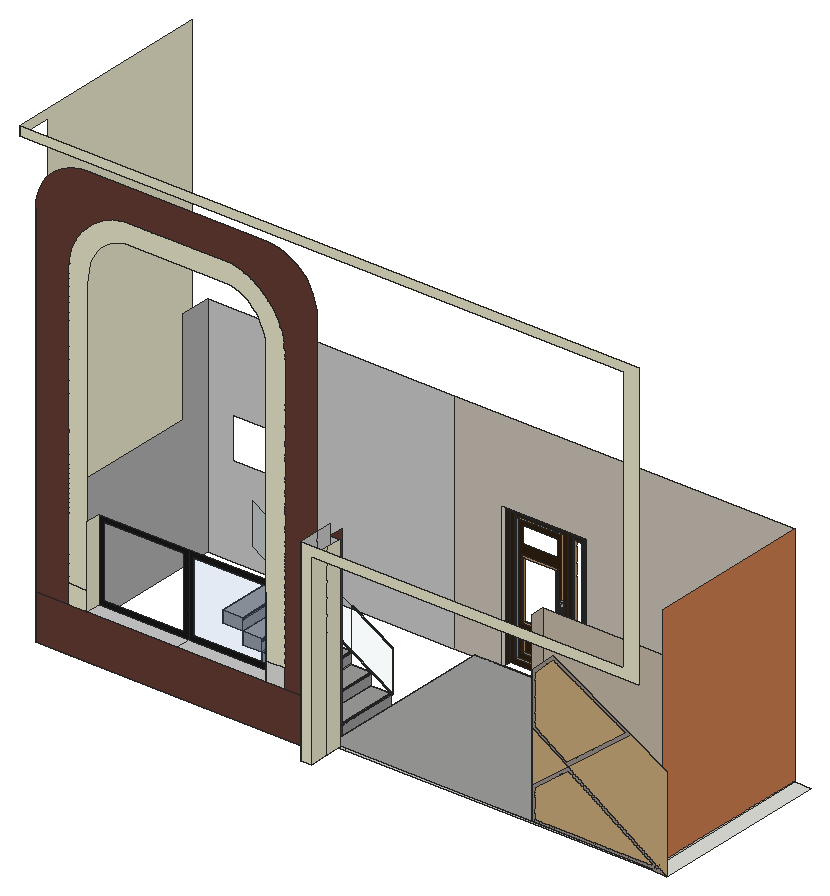
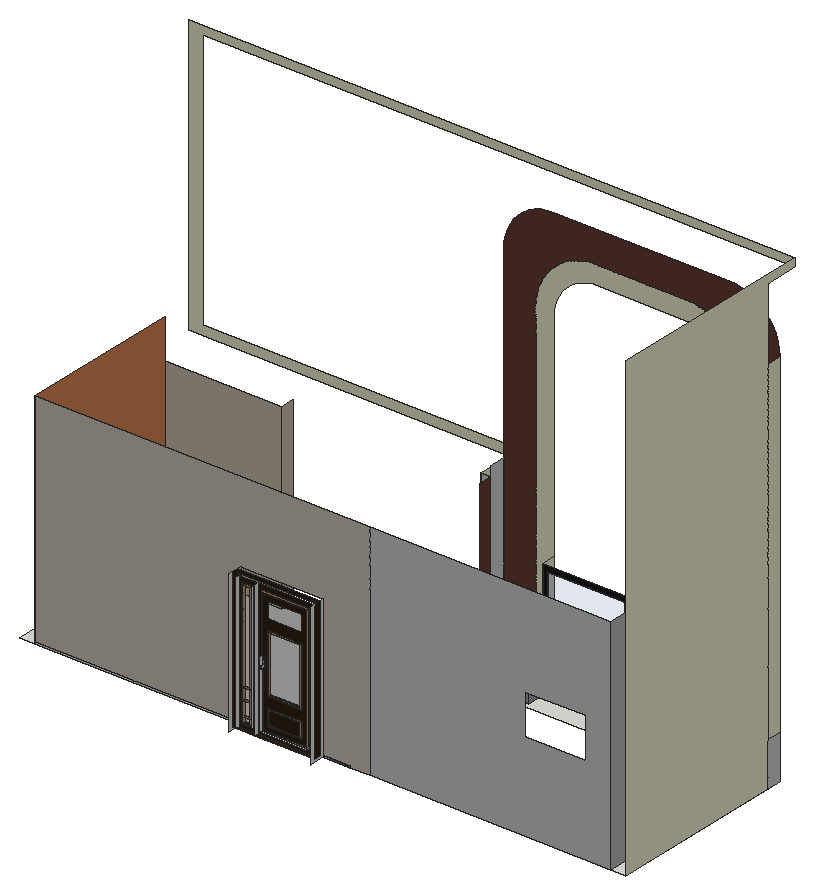
# SketchUp Ruby script. Lengths in inches.
U = 1.inch
M = Sketchup.active_model
def pt(a) = Geom::Point3d.new(a.map { |v| v * U })
def face(e, loops, mat)
  f = e.add_face(loops[0].map { |a| pt(a) })
  loops[1..].each { |l| e.add_face(l.map { |a| pt(a) }).erase! }
  f.material = f.back_material = mat if mat
  f
end
# faces: each face lists its corners as indices into pts; further lists are holes
def faces(e, pts, list, mat = nil) = list.each { |f| face(e, (f[0].is_a?(Array) ? f : [f]).map { |l| l.map { |i| pts[i] } }, mat) }
# xy, xz, yz: faces in a plane at the given z, y or x. An outline is a flat list of corners, or four numbers for a rectangle; further outlines are holes
def ring(l) = l.size == 4 ? [[l[0], l[1]], [l[2], l[1]], [l[2], l[3]], [l[0], l[3]]] : l.each_slice(2).to_a
def flat(e, list, mat, &to3) = list.each { |f| face(e, (f[0].is_a?(Array) ? f : [f]).map { |l| ring(l).map { |u, v| to3.(u, v) } }, mat) }
def xy(e, z, list, mat = nil) = flat(e, list, mat) { |x, y| [x, y, z] }
def xz(e, y, list, mat = nil) = flat(e, list, mat) { |x, z| [x, y, z] }
def yz(e, x, list, mat = nil) = flat(e, list, mat) { |y, z| [x, y, z] }
def lines(e, pts, list) = list.each { |a, b| e.add_line(pt(pts[a]), pt(pts[b])) }
# prism: a flat outline (further loops are holes) pulled along v
def prism(e, loops, v, mat = nil)
  f = face(e, loops, mat); d = Geom::Vector3d.new(v.map { |x| x * U })
  f.pushpull(f.normal.samedirection?(d) ? d.length : -d.length)
end
def box(e, o, s, mat = nil) = prism(e, [[o, [o[0] + s[0], o[1], o[2]], [o[0] + s[0], o[1] + s[1], o[2]], [o[0], o[1] + s[1], o[2]]]], [0, 0, s[2]], mat)
def at(x, y, z, deg = 0) = Geom::Transformation.translation(pt([x, y, z])) * Geom::Transformation.rotation(ORIGIN, Z_AXIS, deg.degrees)
def axes(o, x, y, z) = Geom::Transformation.new([*x, 0, *y, 0, *z, 0, *pt(o).to_a, 1])
def part(name) = M.definitions.add(name)
# library, detail: a bought-in or finely detailed component or shape, given as its bounding box
def library(name, o, s) = part(name).tap { |d| box(d.entities, o, s) }
def detail(e, o, s) = box(e.add_group.entities, o, s)
def put(e, d, t, mat = nil) = e.add_instance(d, t).tap { |i| i.material = mat if mat }
def group(e, t, mat = nil) = e.add_group.tap { |g| g.transformation = t; g.material = mat if mat }.entities
root = M.entities
M.materials.add("Distressed Leather (CCZUWY)").color = [102, 60, 53]
M.materials.add("Drag Textured Plaster None 1500 x 1662 mm (I93S2X)").color = [206, 173, 125]
M.materials.add("Lily_Blonde").color = [237, 233, 206]
M.materials.add("Lily_Light").color = [209, 128, 82]
M.materials.add("Panel-Opening1").color = [191, 148, 107]
M.materials.add("Slate Staggered (K2IBU2)").color = [87, 93, 94]
M.materials.add("Stained Mahogany").color = [48, 33, 18]
M.materials.add("Textured Stucco (8DUEUS)").color = [204, 204, 204]
M.materials.add("Weathered Limestone, Ashlar (46JPNJ)").color = [203, 196, 185]
M.materials.add("Wood Wool (CH8A6D)").color = [158, 148, 138]
M.materials.add("[0136_Charcoal]").color = [25, 25, 25]
M.materials.add("[Aluminum]").color = [178, 178, 178]
M.materials.add("[Metal Rusted]").color = [181, 73, 64]
M.materials.add("[Translucent Glass Blue]1").color = [97, 145, 232]
M.materials["[Translucent Glass Blue]1"].alpha = 0.15
M.materials.add("[Translucent Glass Gray]").color = [73, 161, 170]
M.materials["[Translucent Glass Gray]"].alpha = 0.06
M.materials.add("chiselled-plaster-1800-mm-architextures").color = [198, 187, 169]
M.materials.add("crushed-stone-asphalt-staggered-isosceles-2423-mm-architextu").color = [158, 158, 157]
c1 = part("Stair tread")
xy(c1.entities,0,[[0,0,11.5,36]])
xy(c1.entities,7,[[0,0,11.5,36]])
xz(c1.entities,0,[[0,0,11.5,7],[11.5,6,11.63,6.02,11.75,6.07,11.85,6.15,11.93,6.25,11.98,6.37,12,6.5,11.98,6.63,11.93,6.75,11.85,6.85,11.75,6.93,11.63,6.98,11.5,7]])
xz(c1.entities,36,[[0,0,11.5,7],[11.5,6,11.5,7,11.63,6.98,11.75,6.93,11.85,6.85,11.93,6.75,11.98,6.63,12,6.5,11.98,6.37,11.93,6.25,11.85,6.15,11.75,6.07,11.63,6.02]])
yz(c1.entities,0,[[0,0,36,7]])
yz(c1.entities,11.5,[[0,0,36,6],[0,6,10.3125,7],[10.3125,6,36,7]])
p = [[11.5,36,6],[11.63,36,6.02],[11.63,0,6.02],[11.5,0,6],[11.5,10.3125,6],[11.75,36,6.07],
  [11.75,0,6.07],[11.85,36,6.15],[11.85,0,6.15],[11.93,36,6.25],[11.93,0,6.25],[11.98,36,6.37],
  [11.98,0,6.37],[12,36,6.5],[12,0,6.5],[11.98,36,6.63],[11.98,0,6.63],[11.93,36,6.75],
  [11.93,0,6.75],[11.85,36,6.85],[11.85,0,6.85],[11.75,36,6.93],[11.63,36,6.98],[11.63,0,6.98],
  [11.75,0,6.93],[11.5,36,7],[11.5,10.3125,7],[11.5,0,7]]
faces(c1.entities,p,[[0,1,2,3,4],[1,5,6,2],[5,7,8,6],[7,9,10,8],[9,11,12,10],[11,13,14,12],[13,15,16,14],[15,17,18,16],
  [17,19,20,18],[21,22,23,24],[19,21,24,20],[25,26,27,23,22]])
xy(root,24,[[0,11.4375,9,125.1875],[9,11.4375,163.707,29.1875],[351,20.75,360,125.1875]])
xy(root,24.4375,[[163.707,0,169.707,20.75]],"Textured Stucco (8DUEUS)")
xy(root,25,[[281.1875,20.75,351,29.1875]],"chiselled-plaster-1800-mm-architextures")
xy(root,25,[[164.278,20.75,164.278,125.1875,351,125.1875,351,29.1875,281.1875,29.1875,281.1875,20.75]],"crushed-stone-asphalt-staggered-isosceles-2423-mm-architextu")
xy(root,25.502,[[180.027,127.411,181.898,131.153],[226.808,127.411,228.68,131.153],[181.898,129.282,215.581,131.153],[215.581,129.282,226.808,131.153]],"Stained Mahogany")
xy(root,28.183,[[184.518,129.656,212.961,131.153],[218.2,129.656,224.188,130.405]])
xy(root,28.183,[[184.518,129.282,212.961,129.656],[218.2,129.282,224.188,129.656]],"Stained Mahogany")
xy(root,29.332,[[185.641,129.656,211.838,130.031],[219.323,129.656,223.066,130.592]],"Panel-Opening1")
xy(root,32.204,[[188.447,129.656,209.031,130.031]],"Panel-Opening1")
xy(root,33.353,[[189.57,129.656,207.909,130.405]],"Panel-Opening1")
xy(root,41.012,[[189.57,129.656,207.909,130.405]],"Panel-Opening1")
xy(root,42.161,[[188.447,129.656,209.031,130.031]],"Panel-Opening1")
xy(root,47.905,[[188.447,129.656,209.031,130.031]],"Panel-Opening1")
xy(root,49.054,[[189.57,129.656,207.909,130.405]],"Panel-Opening1")
xy(root,50.0625,[[30,11.4375,81.854,20.1875],[81.854,11.4375,133.707,20.1875]],"Textured Stucco (8DUEUS)")
xy(root,61.961,[[210.464,129.282,212.961,129.282,212.961,129.656,211.838,129.656,211.838,130.031,210.464,130.031]],"[Aluminum]")
xy(root,62.37,[[211.693,129.282,211.713,131.528],[211.713,129.282,211.733,131.528]])
xy(root,62.37,[[211.693,129.095,211.713,129.282],[211.713,129.095,211.733,129.282]],"[Aluminum]")
xy(root,62.916,[[211.652,129.095,211.773,131.715]],"[Metal Rusted]")
xz(root,0,[[163.707,24.4375,169.707,24.4375,169.707,132.8125,360,132.8125,360,298,0,298,0,293,351.576,293,351.576,138.8125,163.707,138.8125]],"Lily_Blonde")
xz(root,11.4375,[[133.707,50.0625,144.724,61.079]])
xz(root,11.4375,[[0,24,163.707,50.0625],[0,50.0625,18.984,50.0625,18.984,220.434,19.341,224.967,19.731,229.931,21.096,235.619,23.334,241.024,26.39,246.011,30.188,250.459,34.636,254.258,39.624,257.314,45.029,259.552,51.14,261.018,113.215,261.018,119.326,259.552,124.731,257.314,129.719,254.258,134.167,250.459,137.966,246.011,141.022,241.024,143.259,235.619,144.624,229.931,145.082,224.1,144.724,219.566,144.724,50.0625,163.707,50.0625,163.707,250,163.451,253.916,162.685,257.765,161.424,261.481,159.688,265,157.508,268.263,154.921,271.213,151.97,273.801,148.707,275.981,145.188,277.716,141.472,278.978,137.623,279.743,133.707,280,30,280,26.084,279.743,22.235,278.978,18.519,277.716,15,275.981,11.737,273.801,8.787,271.213,6.199,268.263,4.019,265,2.284,261.481,1.022,257.765,0.257,253.916,0,250]],"Distressed Leather (CCZUWY)")
xz(root,11.4375,[[18.984,50.0625,30,61.079],[18.984,61.079,30,61.079,30,220,30.324,224.102,30.646,228.204,31.606,232.206,33.18,236.008,35.33,239.517,38.002,242.646,41.131,245.318,44.64,247.468,48.442,249.042,52.443,250.002,111.912,250.002,115.913,249.042,119.715,247.468,123.224,245.318,126.353,242.646,129.025,239.517,131.175,236.008,132.749,232.206,133.709,228.204,134.031,224.102,133.707,220,133.707,61.079,144.724,61.079,144.724,219.566,145.082,224.1,144.624,229.931,143.259,235.619,141.022,241.024,137.966,246.011,134.167,250.459,129.719,254.258,124.731,257.314,119.326,259.552,113.215,261.018,51.14,261.018,45.029,259.552,39.624,257.314,34.636,254.258,30.188,250.459,26.39,246.011,23.334,241.024,21.096,235.619,19.731,229.931,19.341,224.967,18.984,220.434]],"Lily_Blonde")
xz(root,20.1875,[[[30,50.0625,81.854,97.031],[32.83,52.893,79.024,94.201]],[[81.854,50.0625,133.707,97.031],[85.05,53.259,130.511,93.835]]],"[0136_Charcoal]")
xz(root,20.1875,[[85.05,53.259,130.511,93.835]],"[Translucent Glass Blue]1")
xz(root,20.75,[[164.278,24,164.278,24.4375,169.707,24.4375,169.707,25,351,25,351,24],[164.278,24.4375,169.707,25]])
xz(root,20.75,[[360,24,360,78.487,338.67,90.424,301.952,60.664],[352.588,25.588,354.513,25.588,302.067,58.714,282.775,43.077,282.775,26.588,352.588,26.588],[281.1875,43.834,301.952,60.664,281.1875,73.78],[301.832,62.706,335.718,90.171,293.715,113.677,282.85,103.027,282.85,74.696]],"Drag Textured Plaster None 1500 x 1662 mm (I93S2X)")
xz(root,20.75,[[163.707,24.4375,163.707,132.6875,169.707,132.6875,169.707,25,164.278,25,164.278,24.4375]],"Textured Stucco (8DUEUS)")
xz(root,20.75,[[[351,24,360,24,301.952,60.664,281.1875,43.834,281.1875,25,351,25],[352.588,25.588,352.588,26.588,282.775,26.588,282.775,43.077,302.067,58.714,354.513,25.588]],[[301.952,60.664,338.67,90.424,293.441,115.736,281.1875,103.725,281.1875,73.78],[301.832,62.706,282.85,74.696,282.85,103.027,293.715,113.677,335.718,90.171]]],"Wood Wool (CH8A6D)")
xz(root,29.1875,[[281.1875,25,351,132.6875]],"chiselled-plaster-1800-mm-architextures")
xz(root,64.6875,[[164.945,31,164.945,55,141.275,68.956,141.275,44.956],[141.275,44.956,141.275,68.956,118.068,82.639,118.068,58.639],[118.068,58.639,118.068,82.639,83.482,103.25,83.482,79.25,94.982,72.25]],"[Translucent Glass Gray]")
xz(root,125.1875,[[176,24,180.027,25],[180.027,24,229,25],[229,24,230,25],[230,24,351,25]])
xz(root,125.1875,[[164.278,24,176,25]],"Slate Staggered (K2IBU2)")
xz(root,125.1875,[[[9,24,152.42,156],[24,77,60,101]]],"Textured Stucco (8DUEUS)")
xz(root,125.1875,[[152.42,24,164.278,24,164.278,25,180.027,25,180.027,108,229,108,229,25,351,25,351,156,152.42,156]],"Weathered Limestone, Ashlar (46JPNJ)")
xz(root,127.411,[[180.027,25.502,180.027,107.838,228.68,107.838,228.68,25.502,226.808,25.502,226.808,105.923,181.898,105.923,181.898,25.502]],"Stained Mahogany")
xz(root,129.095,[[[211.693,62.37,211.673,62.372,211.633,62.38,211.614,62.386,211.595,62.394,211.577,62.402,211.559,62.412,211.542,62.423,211.526,62.435,211.51,62.448,211.495,62.462,211.482,62.477,211.469,62.493,211.457,62.509,211.437,62.545,211.429,62.564,211.422,62.583,211.416,62.603,211.411,62.623,211.408,62.643,211.406,62.664,211.405,62.684,211.405,64.101,211.406,64.122,211.408,64.142,211.411,64.163,211.416,64.183,211.422,64.203,211.429,64.222,211.437,64.241,211.447,64.259,211.457,64.276,211.469,64.293,211.482,64.309,211.495,64.324,211.51,64.338,211.526,64.351,211.542,64.363,211.559,64.374,211.595,64.392,211.614,64.399,211.633,64.405,211.653,64.41,211.673,64.413,211.693,64.415,211.713,64.416,211.733,64.415,211.753,64.413,211.773,64.41,211.792,64.405,211.811,64.399,211.83,64.392,211.838,64.388,211.849,64.383,211.866,64.374,211.883,64.363,211.9,64.351,211.915,64.338,211.93,64.324,211.944,64.309,211.956,64.293,211.968,64.276,211.979,64.259,211.988,64.241,211.997,64.222,212.004,64.203,212.014,64.163,212.017,64.142,212.019,64.122,212.02,64.101,212.02,62.684,212.019,62.664,212.017,62.643,212.014,62.623,212.004,62.583,211.997,62.564,211.988,62.545,211.979,62.527,211.968,62.509,211.944,62.477,211.93,62.462,211.915,62.448,211.9,62.435,211.883,62.423,211.866,62.412,211.849,62.402,211.838,62.397,211.83,62.394,211.811,62.386,211.792,62.38,211.773,62.376,211.753,62.372,211.733,62.37],[211.652,62.916,211.773,62.916,211.773,64.105,211.772,64.109,211.772,64.113,211.77,64.121,211.768,64.125,211.767,64.128,211.765,64.132,211.763,64.135,211.761,64.139,211.75,64.15,211.746,64.152,211.743,64.154,211.739,64.156,211.736,64.158,211.732,64.159,211.728,64.161,211.724,64.162,211.721,64.162,211.717,64.163,211.709,64.163,211.705,64.162,211.701,64.162,211.697,64.161,211.693,64.159,211.689,64.158,211.686,64.156,211.682,64.154,211.676,64.15,211.673,64.147,211.67,64.145,211.667,64.142,211.665,64.139,211.662,64.135,211.66,64.132,211.658,64.128,211.657,64.125,211.655,64.121,211.653,64.113,211.653,64.109,211.652,64.105]]],"[Metal Rusted]")
xz(root,129.282,[[[181.898,25.502,215.581,105.923],[184.518,28.183,212.961,103.242]],[[215.581,25.502,226.808,105.923],[218.2,28.183,224.188,103.242]]],"Stained Mahogany")
xz(root,129.282,[[[210.464,61.961,212.961,68.107],[211.713,65.58,211.776,65.583,211.838,65.589,211.9,65.599,211.961,65.614,212.022,65.633,212.081,65.655,212.138,65.682,212.193,65.712,212.247,65.746,212.298,65.784,212.347,65.825,212.392,65.869,212.435,65.916,212.475,65.965,212.512,66.018,212.545,66.072,212.575,66.129,212.601,66.188,212.623,66.248,212.641,66.31,212.656,66.372,212.666,66.436,212.672,66.5,212.674,66.564,212.672,66.629,212.666,66.693,212.656,66.756,212.641,66.819,212.623,66.88,212.601,66.941,212.575,66.999,212.545,67.056,212.512,67.111,212.475,67.163,212.435,67.213,212.392,67.26,212.347,67.304,212.298,67.345,212.247,67.382,212.193,67.416,212.138,67.447,212.081,67.473,212.022,67.496,211.961,67.514,211.9,67.529,211.838,67.54,211.776,67.546,211.713,67.548,211.65,67.546,211.587,67.54,211.525,67.529,211.464,67.514,211.404,67.496,211.345,67.473,211.287,67.447,211.232,67.416,211.179,67.382,211.127,67.345,211.079,67.304,211.033,67.26,210.99,67.213,210.95,67.163,210.913,67.111,210.88,67.056,210.85,66.999,210.824,66.941,210.802,66.88,210.784,66.819,210.77,66.756,210.759,66.693,210.753,66.629,210.751,66.564,210.753,66.5,210.759,66.436,210.77,66.372,210.784,66.31,210.802,66.248,210.824,66.188,210.85,66.129,210.88,66.072,210.913,66.018,210.95,65.965,210.99,65.916,211.033,65.869,211.079,65.825,211.127,65.784,211.179,65.746,211.232,65.712,211.287,65.682,211.345,65.655,211.404,65.633,211.464,65.614,211.525,65.599,211.587,65.589,211.65,65.583],[211.693,62.37,211.733,62.37,211.753,62.372,211.773,62.376,211.792,62.38,211.811,62.386,211.83,62.394,211.838,62.397,211.849,62.402,211.866,62.412,211.883,62.423,211.9,62.435,211.915,62.448,211.93,62.462,211.944,62.477,211.968,62.509,211.979,62.527,211.988,62.545,211.997,62.564,212.004,62.583,212.014,62.623,212.017,62.643,212.019,62.664,212.02,62.684,212.02,64.101,212.019,64.122,212.017,64.142,212.014,64.163,212.004,64.203,211.997,64.222,211.988,64.241,211.979,64.259,211.968,64.276,211.956,64.293,211.944,64.309,211.93,64.324,211.915,64.338,211.9,64.351,211.883,64.363,211.866,64.374,211.849,64.383,211.838,64.388,211.83,64.392,211.811,64.399,211.792,64.405,211.773,64.41,211.753,64.413,211.733,64.415,211.713,64.416,211.693,64.415,211.673,64.413,211.653,64.41,211.633,64.405,211.614,64.399,211.595,64.392,211.559,64.374,211.542,64.363,211.526,64.351,211.51,64.338,211.495,64.324,211.482,64.309,211.469,64.293,211.457,64.276,211.447,64.259,211.437,64.241,211.429,64.222,211.422,64.203,211.416,64.183,211.411,64.163,211.408,64.142,211.406,64.122,211.405,64.101,211.405,62.684,211.406,62.664,211.408,62.643,211.411,62.623,211.416,62.603,211.422,62.583,211.429,62.564,211.437,62.545,211.457,62.509,211.469,62.493,211.482,62.477,211.495,62.462,211.51,62.448,211.526,62.435,211.542,62.423,211.559,62.412,211.577,62.402,211.595,62.394,211.614,62.386,211.633,62.38,211.673,62.372]]],"[Aluminum]")
xz(root,129.656,[[184.518,28.183,184.518,103.242,212.961,103.242,212.961,68.107,211.838,68.107,211.838,102.093,185.641,102.093,185.641,29.332,211.838,29.332,211.838,61.961,212.961,61.961,212.961,28.183],[[218.2,28.183,224.188,103.242],[219.323,29.332,223.066,102.093]],[[188.447,32.204,209.031,42.161],[189.57,33.353,207.909,41.012]],[[188.447,47.905,209.031,83.52],[189.57,49.054,207.909,82.371]]],"Panel-Opening1")
xz(root,130.031,[[219.323,32.204,223.066,33.353],[219.323,41.012,223.066,42.135],[219.323,47.905,223.066,49.054]],"Panel-Opening1")
xz(root,130.031,[[[185.641,29.332,185.641,102.093,211.838,102.093,211.838,68.107,210.464,68.107,210.464,61.961,211.838,61.961,211.838,29.332],[188.447,47.905,209.031,83.52],[188.447,89.264,209.031,99.221],[188.447,32.204,209.031,42.161]]],"Stained Mahogany")
xz(root,130.405,[[189.57,33.353,207.909,41.012]],"Stained Mahogany")
yz(root,0,[[20.1875,24,20.1875,293,0,293,0,298,125.1875,298,125.1875,24],[11.4375,50.0625,20.1875,250]],"Lily_Blonde")
yz(root,0,[[11.4375,24,20.1875,50.0625]],"Textured Stucco (8DUEUS)")
yz(root,9,[[29.1875,24,125.1875,24,125.1875,156,107.1875,156,107.1875,101.017,29.1875,101.017]],"[Aluminum]")
yz(root,30,[[11.4375,50.0625,20.1875,97.031]],"Lily_Blonde")
yz(root,133.707,[[11.4375,50.0625,20.1875,97.031]],"Lily_Blonde")
yz(root,163.707,[[11.4375,24,29.1875,24,29.1875,132.6875,20.75,132.6875,20.75,24.4375,11.4375,24.4375]],"Distressed Leather (CCZUWY)")
yz(root,163.707,[[0,24.4375,11.4375,138.8125],[11.4375,24.4375,20.75,138.8125]],"Textured Stucco (8DUEUS)")
yz(root,164.278,[[20.75,24,125.1875,25]])
yz(root,164.945,[[64.6875,31,65.1875,55]])
yz(root,169.707,[[0,24.4375,11.4375,132.8125],[11.4375,24.4375,20.75,132.8125]],"Lily_Blonde")
yz(root,180.027,[[[125.1875,24,134.1875,108],[127.411,25.502,131.153,107.838]]])
yz(root,180.027,[[127.411,25.502,131.153,107.838]],"Stained Mahogany")
yz(root,181.898,[[129.282,25.502,131.153,105.923]])
yz(root,181.898,[[127.411,25.502,129.282,105.923]],"Stained Mahogany")
yz(root,184.518,[[129.282,28.183,129.656,103.242]],"Stained Mahogany")
yz(root,185.641,[[129.656,29.332,130.031,102.093]],"Panel-Opening1")
yz(root,188.447,[[129.656,32.204,130.031,42.161],[129.656,47.905,130.031,83.52]],"Panel-Opening1")
yz(root,189.57,[[129.656,33.353,130.405,41.012],[129.656,49.054,130.405,82.371]],"Panel-Opening1")
yz(root,207.909,[[129.656,33.353,130.405,41.012],[129.656,49.054,130.405,82.371]],"Panel-Opening1")
yz(root,209.031,[[129.656,32.204,130.031,42.161],[129.656,47.905,130.031,83.52]],"Panel-Opening1")
yz(root,210.464,[[129.282,61.961,130.031,68.107]],"[Aluminum]")
yz(root,211.405,[[129.282,62.684,131.528,64.101]])
yz(root,211.405,[[129.095,62.684,129.282,64.101]],"[Aluminum]")
yz(root,211.652,[[129.095,62.916,131.715,64.097],[129.095,64.097,131.715,64.105]],"[Metal Rusted]")
yz(root,211.653,[[129.095,64.109,131.715,64.113]],"[Metal Rusted]")
yz(root,211.772,[[129.095,64.109,131.715,64.113]],"[Metal Rusted]")
yz(root,211.773,[[129.095,62.916,131.715,64.097],[129.095,64.097,131.715,64.105]],"[Metal Rusted]")
yz(root,211.838,[[129.656,29.332,130.031,61.961]],"Panel-Opening1")
yz(root,212.02,[[129.282,62.684,131.528,64.101]])
yz(root,212.02,[[129.095,62.684,129.282,64.101]],"[Aluminum]")
yz(root,212.961,[[129.656,28.183,131.153,61.961],[129.282,61.961,131.153,68.107]])
yz(root,212.961,[[129.282,28.183,129.656,61.961]],"Stained Mahogany")
yz(root,215.581,[[129.282,25.502,131.153,105.923]])
yz(root,218.2,[[129.656,28.183,130.405,103.242]])
yz(root,218.2,[[129.282,28.183,129.656,103.242]],"Stained Mahogany")
yz(root,219.323,[[130.031,32.204,130.592,33.353],[130.031,41.012,130.592,42.135],[130.031,47.905,130.592,49.054]])
yz(root,219.323,[[129.656,29.332,130.592,29.332,130.592,32.204,130.031,32.204,130.031,33.353,130.592,33.353,130.592,41.012,130.031,41.012,130.031,42.135,130.592,42.135,130.592,47.905,130.031,47.905,130.031,49.054,130.592,49.054,130.592,82.371,130.031,82.371,130.031,83.52,130.592,83.52,130.592,89.264,130.031,89.264,130.031,90.413,130.592,90.413,130.592,98.072,130.031,98.072,130.031,99.221,130.592,99.221,130.592,102.093,129.656,102.093]],"Panel-Opening1")
yz(root,223.066,[[130.031,32.204,130.592,33.353],[130.031,41.012,130.592,42.135],[130.031,47.905,130.592,49.054]])
yz(root,223.066,[[129.656,29.332,129.656,102.093,130.592,102.093,130.592,99.221,130.031,99.221,130.031,98.072,130.592,98.072,130.592,90.413,130.031,90.413,130.031,89.264,130.592,89.264,130.592,83.52,130.031,83.52,130.031,82.371,130.592,82.371,130.592,49.054,130.031,49.054,130.031,47.905,130.592,47.905,130.592,42.135,130.031,42.135,130.031,41.012,130.592,41.012,130.592,33.353,130.031,33.353,130.031,32.204,130.592,32.204,130.592,29.332]],"Panel-Opening1")
yz(root,224.188,[[129.656,28.183,130.405,103.242]])
yz(root,224.188,[[129.282,28.183,129.656,103.242]],"Stained Mahogany")
yz(root,226.808,[[129.282,25.502,131.153,105.923]])
yz(root,226.808,[[127.411,25.502,129.282,105.923]],"Stained Mahogany")
yz(root,228.68,[[127.411,25.502,131.153,107.838]],"Stained Mahogany")
yz(root,229,[[125.1875,24,134.1875,108]])
yz(root,281.1875,[[20.75,25,29.1875,132.6875]],"chiselled-plaster-1800-mm-architextures")
yz(root,351,[[20.75,24,29.1875,25],[29.1875,24,125.1875,25]])
yz(root,351,[[29.1875,25,125.1875,156]],"Lily_Light")
p = [[141.275,65.1875,44.956],[164.945,65.1875,31],[164.945,64.6875,31],[141.275,64.6875,44.956],[118.068,65.1875,58.639],[118.068,64.6875,58.639],
  [164.945,65.1875,55],[141.275,65.1875,68.956],[141.275,64.6875,68.956],[164.945,64.6875,55],[94.982,65.1875,72.25],[94.982,64.6875,72.25],
  [211.559,129.282,62.412],[211.542,129.282,62.423],[211.542,129.095,62.423],[211.559,129.095,62.412],[211.526,129.282,62.435],[211.526,129.095,62.435],
  [211.51,129.282,62.448],[211.51,129.095,62.448],[211.495,129.282,62.462],[211.495,129.095,62.462],[211.653,129.282,62.376],[211.633,129.282,62.38],
  [211.633,129.095,62.38],[211.653,129.095,62.376],[211.614,129.282,62.386],[211.614,129.095,62.386],[211.595,129.282,62.394],[211.595,129.095,62.394],
  [211.577,129.282,62.402],[211.577,129.095,62.402],[211.693,129.282,62.37],[211.673,129.282,62.372],[211.673,129.095,62.372],[211.693,129.095,62.37],
  [211.753,129.282,62.372],[211.733,129.282,62.37],[211.733,129.095,62.37],[211.753,129.095,62.372],[211.773,129.282,62.376],[211.773,129.095,62.376],
  [211.792,129.282,62.38],[211.792,129.095,62.38],[211.811,129.282,62.386],[211.811,129.095,62.386],[211.83,129.282,62.394],[211.83,129.095,62.394],
  [211.838,129.282,62.397],[211.838,129.095,62.397],[211.849,129.282,62.402],[211.849,129.095,62.402],[211.866,129.282,62.412],[211.866,129.095,62.412],
  [211.883,129.282,62.423],[211.883,129.095,62.423],[211.9,129.282,62.435],[211.9,129.095,62.435],[211.915,129.282,62.448],[211.915,129.095,62.448],
  [211.93,129.282,62.462],[211.93,129.095,62.462],[211.542,131.528,62.423],[211.526,131.528,62.435],[211.559,131.528,62.412],[211.51,131.528,62.448],
  [211.495,131.528,62.462],[211.653,131.528,62.376],[211.633,131.528,62.38],[211.614,131.528,62.386],[211.595,131.528,62.394],[211.577,131.528,62.402],
  [211.753,131.528,62.372],[211.733,131.528,62.37],[211.693,131.528,62.37],[211.673,131.528,62.372],[211.773,131.528,62.376],[211.792,131.528,62.38],
  [211.811,131.528,62.386],[211.83,131.528,62.394],[211.838,131.528,62.397],[211.849,131.528,62.402],[211.866,131.528,62.412],[211.883,131.528,62.423],
  [211.9,131.528,62.435],[211.915,131.528,62.448],[211.93,131.528,62.462],[211.457,129.282,62.509],[211.447,129.282,62.527],[211.447,129.095,62.527],
  [211.457,129.095,62.509],[211.437,129.282,62.545],[211.437,129.095,62.545],[211.429,129.282,62.564],[211.429,129.095,62.564],[211.482,129.282,62.477],
  [211.482,129.095,62.477],[211.469,129.282,62.493],[211.469,129.095,62.493],[211.944,129.282,62.477],[211.944,129.095,62.477],[211.956,129.282,62.493],
  [211.956,129.095,62.493],[211.968,129.282,62.509],[211.968,129.095,62.509],[211.979,129.282,62.527],[211.979,129.095,62.527],[211.988,129.282,62.545],
  [211.988,129.095,62.545],[211.997,129.282,62.564],[211.997,129.095,62.564],[211.457,131.528,62.509],[211.447,131.528,62.527],[211.437,131.528,62.545],
  [211.429,131.528,62.564],[211.482,131.528,62.477],[211.469,131.528,62.493],[211.944,131.528,62.477],[211.956,131.528,62.493],[211.968,131.528,62.509],
  [211.979,131.528,62.527],[211.988,131.528,62.545],[211.997,131.528,62.564],[211.422,129.282,62.583],[211.422,129.095,62.583],[211.416,129.282,62.603],
  [211.416,129.095,62.603],[211.411,129.282,62.623],[211.411,129.095,62.623],[211.408,129.282,62.643],[211.408,129.095,62.643],[211.406,129.282,62.664],
  [211.406,129.095,62.664],[212.004,129.282,62.583],[212.004,129.095,62.583],[212.009,129.282,62.603],[212.009,129.095,62.603],[212.014,129.282,62.623],
  [212.014,129.095,62.623],[212.017,129.282,62.643],[212.017,129.095,62.643],[212.019,129.282,62.664],[212.019,129.095,62.664],[211.422,131.528,62.583],
  [211.416,131.528,62.603],[211.411,131.528,62.623],[211.408,131.528,62.643],[211.406,131.528,62.664],[212.004,131.528,62.583],[212.009,131.528,62.603],
  [212.014,131.528,62.623],[212.017,131.528,62.643],[212.019,131.528,62.664],[211.405,129.282,62.684],[211.405,129.095,62.684],[212.02,129.282,62.684],
  [212.02,129.095,62.684],[211.405,131.528,62.684],[212.02,131.528,62.684],[211.405,129.282,64.101],[211.406,129.282,64.122],[211.406,129.095,64.122],
  [211.405,129.095,64.101],[211.408,129.282,64.142],[211.408,129.095,64.142],[211.411,129.282,64.163],[211.411,129.095,64.163],[211.652,131.715,64.105],
  [211.652,129.095,64.105],[211.653,129.095,64.109],[211.653,131.715,64.109],[211.653,131.715,64.113],[211.653,129.095,64.113],[211.654,129.095,64.117],
  [211.654,131.715,64.117],[211.655,129.095,64.121],[211.655,131.715,64.121],[211.657,129.095,64.125],[211.657,131.715,64.125],[211.658,129.095,64.128],
  [211.658,131.715,64.128],[211.66,129.095,64.132],[211.66,131.715,64.132],[211.662,129.095,64.135],[211.662,131.715,64.135],[211.665,129.095,64.139],
  [211.665,131.715,64.139],[211.667,129.095,64.142],[211.667,131.715,64.142],[211.67,129.095,64.145],[211.67,131.715,64.145],[211.673,129.095,64.147],
  [211.673,131.715,64.147],[211.676,129.095,64.15],[211.676,131.715,64.15],[211.772,131.715,64.109],[211.772,129.095,64.109],[211.773,129.095,64.105],
  [211.773,131.715,64.105],[211.771,131.715,64.117],[211.771,129.095,64.117],[211.772,129.095,64.113],[211.772,131.715,64.113],[211.77,131.715,64.121],
  [211.77,129.095,64.121],[211.768,131.715,64.125],[211.768,129.095,64.125],[211.767,131.715,64.128],[211.767,129.095,64.128],[211.765,131.715,64.132],
  [211.765,129.095,64.132],[211.763,131.715,64.135],[211.763,129.095,64.135],[211.761,131.715,64.139],[211.761,129.095,64.139],[211.758,131.715,64.142],
  [211.758,129.095,64.142],[211.755,131.715,64.145],[211.755,129.095,64.145],[211.753,131.715,64.147],[211.753,129.095,64.147],[212.019,129.282,64.122],
  [212.02,129.282,64.101],[212.02,129.095,64.101],[212.019,129.095,64.122],[212.017,129.282,64.142],[212.017,129.095,64.142],[212.014,129.282,64.163],
  [212.014,129.095,64.163],[211.405,131.528,64.101],[211.406,131.528,64.122],[211.408,131.528,64.142],[211.411,131.528,64.163],[212.019,131.528,64.122],
  [212.02,131.528,64.101],[212.017,131.528,64.142],[212.014,131.528,64.163],[211.416,129.282,64.183],[211.416,129.095,64.183],[211.422,129.282,64.203],
  [211.422,129.095,64.203],[211.429,129.282,64.222],[211.429,129.095,64.222],[211.437,129.282,64.241],[211.437,129.095,64.241],[211.447,129.282,64.259],
  [211.447,129.095,64.259],[212.009,129.282,64.183],[212.009,129.095,64.183],[212.004,129.282,64.203],[212.004,129.095,64.203],[211.997,129.282,64.222],
  [211.997,129.095,64.222],[211.988,129.282,64.241],[211.988,129.095,64.241],[211.979,129.282,64.259],[211.979,129.095,64.259],[211.457,129.282,64.276],
  [211.457,129.095,64.276],[211.469,129.282,64.293],[211.469,129.095,64.293],[211.482,129.282,64.309],[211.482,129.095,64.309],[211.495,129.282,64.324],
  [211.495,129.095,64.324],[211.51,129.282,64.338],[211.51,129.095,64.338],[211.526,129.282,64.351],[211.526,129.095,64.351],[211.944,129.282,64.309],
  [211.956,129.282,64.293],[211.956,129.095,64.293],[211.944,129.095,64.309],[211.93,129.282,64.324],[211.93,129.095,64.324],[211.915,129.282,64.338],
  [211.915,129.095,64.338],[211.9,129.282,64.351],[211.9,129.095,64.351],[211.968,129.282,64.276],[211.968,129.095,64.276],[211.542,129.282,64.363],
  [211.542,129.095,64.363],[211.559,129.282,64.374],[211.559,129.095,64.374],[211.577,129.282,64.383],[211.577,129.095,64.383],[211.595,129.282,64.392],
  [211.595,129.095,64.392],[211.633,129.282,64.405],[211.653,129.282,64.41],[211.653,129.095,64.41],[211.633,129.095,64.405],[211.614,129.282,64.399],
  [211.614,129.095,64.399],[211.693,129.282,64.415],[211.713,129.282,64.416],[211.713,129.095,64.416],[211.693,129.095,64.415],[211.673,129.282,64.413],
  [211.673,129.095,64.413],[211.733,129.282,64.415],[211.753,129.282,64.413],[211.753,129.095,64.413],[211.733,129.095,64.415],[211.849,129.282,64.383],
  [211.866,129.282,64.374],[211.866,129.095,64.374],[211.849,129.095,64.383],[211.838,129.282,64.388],[211.838,129.095,64.388],[211.811,129.282,64.399],
  [211.83,129.282,64.392],[211.83,129.095,64.392],[211.811,129.095,64.399],[211.773,129.282,64.41],[211.773,129.095,64.41],[211.792,129.282,64.405],
  [211.792,129.095,64.405],[211.883,129.282,64.363],[211.883,129.095,64.363],[355.402,20.75,28.402],[355.598,20.75,28.402]]
faces(root,p,[[0,1,2,3],[4,0,3,5],[6,7,8,9],[10,4,5,11],[62,13,16,63],[64,12,13,62],[63,16,18,65],[65,18,20,66],
  [67,22,23,68],[68,23,26,69],[69,26,28,70],[70,28,30,71],[71,30,12,64],[72,36,37,73],[74,32,33,75],[75,33,22,67],
  [76,40,36,72],[77,42,40,76],[78,44,42,77],[79,46,44,78],[80,48,46,79],[81,50,48,80],[82,52,50,81],[83,54,52,82],
  [84,56,54,83],[85,58,56,84],[86,60,58,85],[111,87,88,112],[112,88,91,113],[113,91,93,114],[66,20,95,115],[115,95,97,116],
  [116,97,87,111],[117,99,60,86],[118,101,99,117],[119,103,101,118],[120,105,103,119],[121,107,105,120],[122,109,107,121],[114,93,123,143],
  [143,123,125,144],[144,125,127,145],[145,127,129,146],[146,129,131,147],[148,133,109,122],[149,135,133,148],[150,137,135,149],[151,139,137,150],
  [152,141,139,151],[147,131,153,157],[158,155,141,152],[229,159,160,230],[230,160,163,231],[231,163,165,232],[233,221,222,234],[235,225,221,233],
  [236,227,225,235]])
faces(root,p,[[12,13,14,15],[13,16,17,14],[16,18,19,17],[18,20,21,19],[22,23,24,25],[23,26,27,24],[26,28,29,27],[28,30,31,29],
  [30,12,15,31],[32,33,34,35],[36,37,38,39],[33,22,25,34],[40,36,39,41],[42,40,41,43],[44,42,43,45],[46,44,45,47],
  [48,46,47,49],[50,48,49,51],[52,50,51,53],[54,52,53,55],[56,54,55,57],[58,56,57,59],[60,58,59,61],[87,88,89,90],
  [88,91,92,89],[91,93,94,92],[20,95,96,21],[95,97,98,96],[97,87,90,98],[99,60,61,100],[101,99,100,102],[103,101,102,104],
  [105,103,104,106],[107,105,106,108],[109,107,108,110],[93,123,124,94],[123,125,126,124],[125,127,128,126],[127,129,130,128],[129,131,132,130],
  [133,109,110,134],[135,133,134,136],[137,135,136,138],[139,137,138,140],[141,139,140,142],[131,153,154,132],[155,141,142,156],[159,160,161,162],
  [160,163,164,161],[163,165,166,164],[221,222,223,224],[225,221,224,226],[227,225,226,228],[165,237,238,166],[237,239,240,238],[239,241,242,240],
  [241,243,244,242],[243,245,246,244],[247,227,228,248],[249,247,248,250],[251,249,250,252],[253,251,252,254],[255,253,254,256],[245,257,258,246],
  [257,259,260,258],[259,261,262,260],[261,263,264,262],[263,265,266,264],[265,267,268,266],[269,270,271,272],[273,269,272,274],[275,273,274,276],
  [277,275,276,278],[279,255,256,280],[270,279,280,271],[267,281,282,268],[281,283,284,282],[283,285,286,284],[285,287,288,286],[289,290,291,292],
  [287,293,294,288],[293,289,292,294],[295,296,297,298],[290,299,300,291],[301,302,303,304],[299,295,298,300],[296,301,304,297],[305,306,307,308],
  [309,305,308,310],[311,312,313,314],[302,315,316,303],[312,309,310,313],[317,311,314,318],[315,317,318,316],[319,277,278,320],[306,319,320,307]],"[Aluminum]")
faces(root,p,[[167,168,169,170],[171,172,173,174],[174,173,175,176],[176,175,177,178],[178,177,179,180],[180,179,181,182],[182,181,183,184],[184,183,185,186],
  [186,185,187,188],[188,187,189,190],[190,189,191,192],[192,191,193,194],[195,196,197,198],[199,200,201,202],[203,204,200,199],[205,206,204,203],
  [207,208,206,205],[209,210,208,207],[211,212,210,209],[213,214,212,211],[215,216,214,213],[217,218,216,215],[219,220,218,217]],"[Metal Rusted]")
lines(root,p,[[321,322]])
put(root,c1,at(152.05,29.1875,24),"crushed-stone-asphalt-staggered-isosceles-2423-mm-architextu")
put(root,c1,at(140.55,29.1875,31),"crushed-stone-asphalt-staggered-isosceles-2423-mm-architextu")
put(root,c1,at(129.05,29.1875,38),"crushed-stone-asphalt-staggered-isosceles-2423-mm-architextu")
put(root,c1,at(117.55,29.1875,45),"crushed-stone-asphalt-staggered-isosceles-2423-mm-architextu")
put(root,c1,at(106.05,29.1875,52),"crushed-stone-asphalt-staggered-isosceles-2423-mm-architextu")
put(root,c1,at(94.55,29.1875,59),"crushed-stone-asphalt-staggered-isosceles-2423-mm-architextu")
